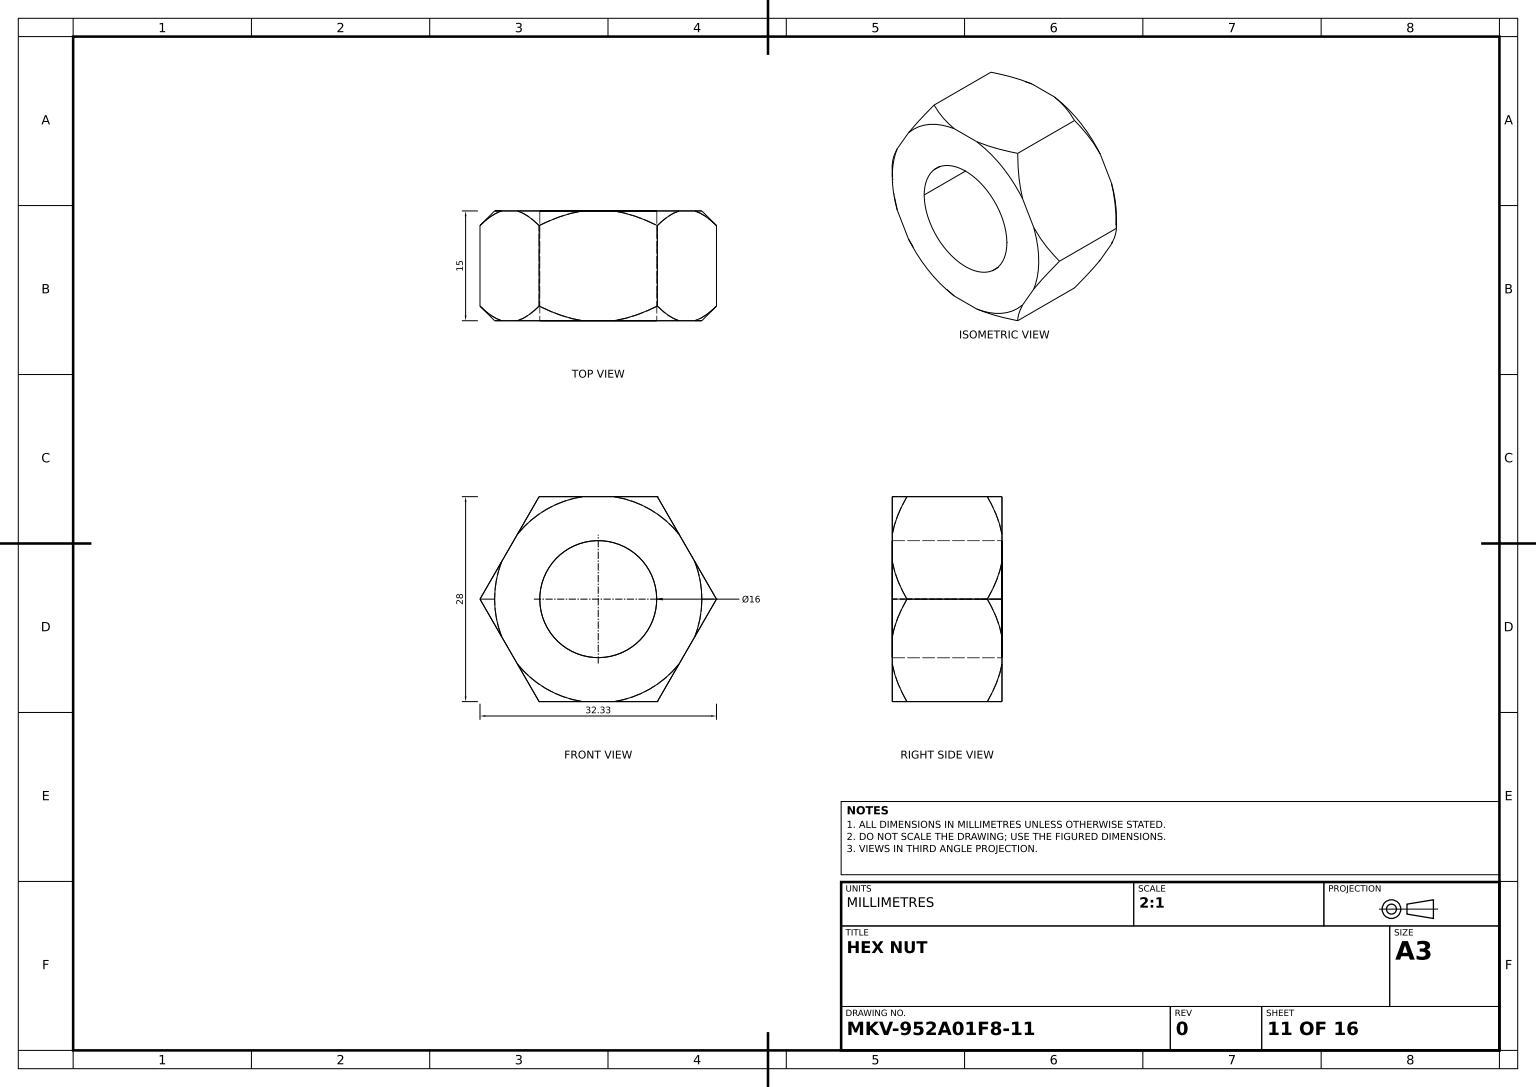
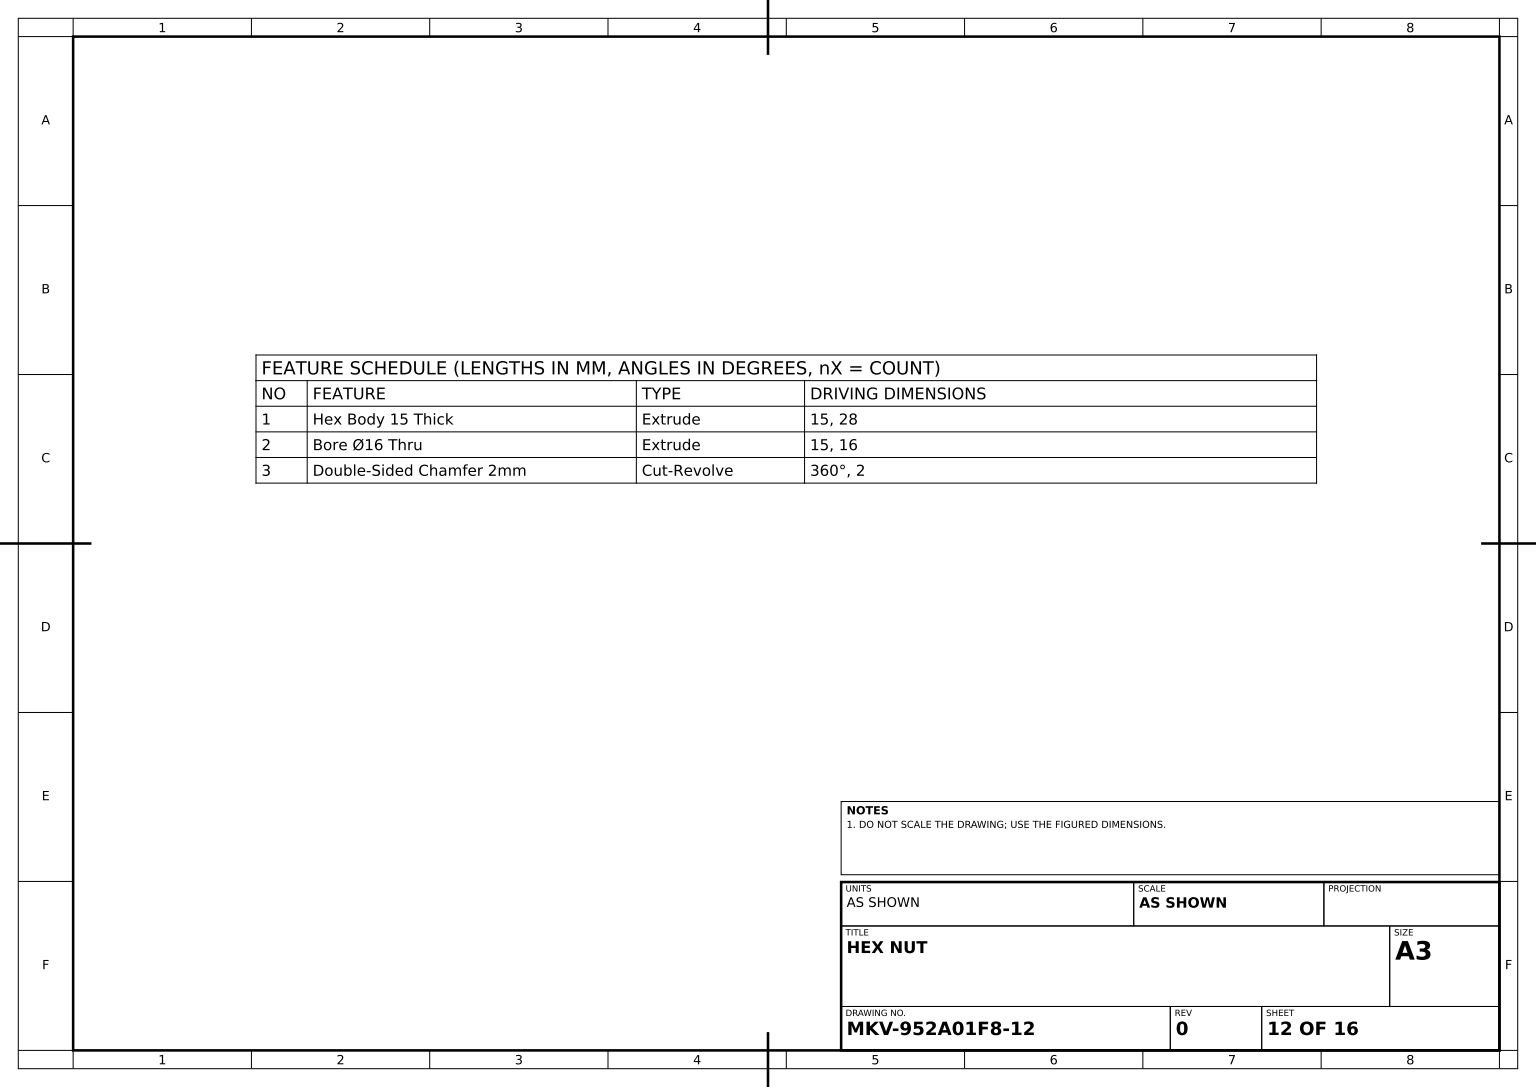
ISO-10303-21;
HEADER;
FILE_DESCRIPTION((''),'2;1');
FILE_NAME('','',(''),(''),'','','');
FILE_SCHEMA(('AUTOMOTIVE_DESIGN'));
ENDSEC;
DATA;
#1=APPLICATION_CONTEXT('');
#2=PRODUCT_CONTEXT('',#1,'mechanical');
#3=PRODUCT('','','',(#2));
#4=PRODUCT_DEFINITION_FORMATION('','',#3);
#5=PRODUCT_DEFINITION_CONTEXT('',#1,'design');
#6=PRODUCT_DEFINITION('','',#4,#5);
#7=PRODUCT_DEFINITION_SHAPE('','',#6);
#8=(LENGTH_UNIT()NAMED_UNIT(*)SI_UNIT(.MILLI.,.METRE.));
#9=(NAMED_UNIT(*)PLANE_ANGLE_UNIT()SI_UNIT($,.RADIAN.));
#10=(NAMED_UNIT(*)SI_UNIT($,.STERADIAN.)SOLID_ANGLE_UNIT());
#11=UNCERTAINTY_MEASURE_WITH_UNIT(LENGTH_MEASURE(1.E-05),#8,'distance_accuracy_value','');
#12=(GEOMETRIC_REPRESENTATION_CONTEXT(3)GLOBAL_UNCERTAINTY_ASSIGNED_CONTEXT((#11))GLOBAL_UNIT_ASSIGNED_CONTEXT((#8,#9,#10))REPRESENTATION_CONTEXT('',''));
#13=CARTESIAN_POINT('',(16.165808,0.,5.5));
#14=VERTEX_POINT('',#13);
#15=CARTESIAN_POINT('',(13.204877,-5.128483,7.5));
#16=VERTEX_POINT('',#15);
#17=CARTESIAN_POINT('',(15.693285,-0.818433,5.972523));
#18=CARTESIAN_POINT('',(15.212718,-1.6508,6.391638));
#19=CARTESIAN_POINT('',(14.228435,-3.355628,7.07619));
#20=CARTESIAN_POINT('',(13.724685,-4.228148,7.341403));
#21=B_SPLINE_CURVE_WITH_KNOTS('',3,(#13,#17,#18,#19,#20,#15),.UNSPECIFIED.,.F.,.F.,(4,2,4),(0.000000891,0.003124417,0.006247943),.UNSPECIFIED.);
#22=EDGE_CURVE('',#14,#16,#21,.T.);
#23=ORIENTED_EDGE('',*,*,#22,.T.);
#24=CARTESIAN_POINT('',(11.043835,-8.871517,7.5));
#25=VERTEX_POINT('',#24);
#26=CARTESIAN_POINT('',(8.082904,-14.,7.5));
#27=DIRECTION('',(0.5,0.866025404,0.));
#28=VECTOR('',#27,1000.);
#29=LINE('',#26,#28);
#30=EDGE_CURVE('',#25,#16,#29,.T.);
#31=ORIENTED_EDGE('',*,*,#30,.F.);
#32=CARTESIAN_POINT('',(8.082904,-14.,5.5));
#33=VERTEX_POINT('',#32);
#34=CARTESIAN_POINT('',(10.787509,-9.315486,7.421793));
#35=CARTESIAN_POINT('',(10.532672,-9.756876,7.316818));
#36=CARTESIAN_POINT('',(10.025695,-10.634987,7.058372));
#37=CARTESIAN_POINT('',(9.773626,-11.071583,6.904751));
#38=CARTESIAN_POINT('',(9.031896,-12.356297,6.388584));
#39=CARTESIAN_POINT('',(8.552376,-13.186851,5.969472));
#40=B_SPLINE_CURVE_WITH_KNOTS('',3,(#24,#34,#35,#36,#37,#38,#39,#32),.UNSPECIFIED.,.F.,.F.,(4,2,2,4),(0.010529143,0.012071736,0.013614329,0.016699514),.UNSPECIFIED.);
#41=EDGE_CURVE('',#25,#33,#40,.T.);
#42=ORIENTED_EDGE('',*,*,#41,.T.);
#43=CARTESIAN_POINT('',(8.082904,-14.,-5.5));
#44=VERTEX_POINT('',#43);
#45=DIRECTION('',(0.,0.,-1.));
#46=VECTOR('',#45,1000.);
#47=LINE('',#26,#46);
#48=EDGE_CURVE('',#33,#44,#47,.T.);
#49=ORIENTED_EDGE('',*,*,#48,.T.);
#50=CARTESIAN_POINT('',(11.043835,-8.871517,-7.5));
#51=VERTEX_POINT('',#50);
#52=CARTESIAN_POINT('',(8.555426,-13.181567,-5.972523));
#53=CARTESIAN_POINT('',(9.035994,-12.3492,-6.391638));
#54=CARTESIAN_POINT('',(10.020277,-10.644372,-7.07619));
#55=CARTESIAN_POINT('',(10.524026,-9.771852,-7.341403));
#56=B_SPLINE_CURVE_WITH_KNOTS('',3,(#43,#52,#53,#54,#55,#50),.UNSPECIFIED.,.F.,.F.,(4,2,4),(0.000000891,0.003124417,0.006247943),.UNSPECIFIED.);
#57=EDGE_CURVE('',#44,#51,#56,.T.);
#58=ORIENTED_EDGE('',*,*,#57,.T.);
#59=CARTESIAN_POINT('',(13.204877,-5.128483,-7.5));
#60=VERTEX_POINT('',#59);
#61=CARTESIAN_POINT('',(8.082904,-14.,-7.5));
#62=LINE('',#61,#28);
#63=EDGE_CURVE('',#51,#60,#62,.T.);
#64=ORIENTED_EDGE('',*,*,#63,.T.);
#65=CARTESIAN_POINT('',(16.165808,0.,-5.5));
#66=VERTEX_POINT('',#65);
#67=CARTESIAN_POINT('',(13.461202,-4.684514,-7.421793));
#68=CARTESIAN_POINT('',(13.716039,-4.243124,-7.316818));
#69=CARTESIAN_POINT('',(14.223016,-3.365013,-7.058372));
#70=CARTESIAN_POINT('',(14.475085,-2.928417,-6.904751));
#71=CARTESIAN_POINT('',(15.216815,-1.643703,-6.388584));
#72=CARTESIAN_POINT('',(15.696336,-0.813149,-5.969472));
#73=B_SPLINE_CURVE_WITH_KNOTS('',3,(#59,#67,#68,#69,#70,#71,#72,#65),.UNSPECIFIED.,.F.,.F.,(4,2,2,4),(0.010529143,0.012071736,0.013614329,0.016699514),.UNSPECIFIED.);
#74=EDGE_CURVE('',#60,#66,#73,.T.);
#75=ORIENTED_EDGE('',*,*,#74,.T.);
#76=CARTESIAN_POINT('',(16.165808,0.,7.5));
#77=LINE('',#76,#46);
#78=EDGE_CURVE('',#14,#66,#77,.T.);
#79=ORIENTED_EDGE('',*,*,#78,.F.);
#80=EDGE_LOOP('',(#23,#31,#42,#49,#58,#64,#75,#79));
#81=FACE_OUTER_BOUND('',#80,.T.);
#82=DIRECTION('',(-0.866025404,0.5,0.));
#83=DIRECTION('',(-0.5,-0.866025404,0.));
#84=AXIS2_PLACEMENT_3D('',#26,#82,#83);
#85=PLANE('',#84);
#86=ADVANCED_FACE('',(#81),#85,.F.);
#87=CARTESIAN_POINT('',(13.204877,5.128483,7.5));
#88=VERTEX_POINT('',#87);
#89=CARTESIAN_POINT('',(13.461202,4.684514,7.421793));
#90=CARTESIAN_POINT('',(13.716039,4.243124,7.316818));
#91=CARTESIAN_POINT('',(14.223016,3.365013,7.058372));
#92=CARTESIAN_POINT('',(14.475085,2.928417,6.904751));
#93=CARTESIAN_POINT('',(15.216815,1.643703,6.388584));
#94=CARTESIAN_POINT('',(15.696336,0.813149,5.969472));
#95=B_SPLINE_CURVE_WITH_KNOTS('',3,(#87,#89,#90,#91,#92,#93,#94,#13),.UNSPECIFIED.,.F.,.F.,(4,2,2,4),(0.010529143,0.012071736,0.013614329,0.016699514),.UNSPECIFIED.);
#96=EDGE_CURVE('',#88,#14,#95,.T.);
#97=ORIENTED_EDGE('',*,*,#96,.F.);
#98=CARTESIAN_POINT('',(0.,0.,7.5));
#99=DIRECTION('',(1.,0.,0.));
#100=AXIS2_PLACEMENT_3D('',#98,#45,#99);
#101=CIRCLE('',#100,14.165808);
#102=EDGE_CURVE('',#88,#16,#101,.T.);
#103=ORIENTED_EDGE('',*,*,#102,.T.);
#104=ORIENTED_EDGE('',*,*,#22,.F.);
#105=EDGE_LOOP('',(#97,#103,#104));
#106=FACE_OUTER_BOUND('',#105,.T.);
#107=CARTESIAN_POINT('',(0.,0.,5.5));
#108=DIRECTION('',(-1.,0.,0.));
#109=AXIS2_PLACEMENT_3D('',#107,#45,#108);
#110=CONICAL_SURFACE('',#109,16.165807537,0.785398163);
#111=ADVANCED_FACE('',(#106),#110,.T.);
#112=CARTESIAN_POINT('',(2.161042,-14.,-7.5));
#113=VERTEX_POINT('',#112);
#114=CARTESIAN_POINT('',(0.,0.,-7.5));
#115=AXIS2_PLACEMENT_3D('',#114,#45,#99);
#116=CIRCLE('',#115,14.165808);
#117=EDGE_CURVE('',#51,#113,#116,.T.);
#118=ORIENTED_EDGE('',*,*,#117,.F.);
#119=ORIENTED_EDGE('',*,*,#57,.F.);
#120=CARTESIAN_POINT('',(2.673693,-14.,-7.421793));
#121=CARTESIAN_POINT('',(3.183366,-14.,-7.316818));
#122=CARTESIAN_POINT('',(4.197321,-14.,-7.058372));
#123=CARTESIAN_POINT('',(4.701458,-14.,-6.904751));
#124=CARTESIAN_POINT('',(6.184918,-14.,-6.388584));
#125=CARTESIAN_POINT('',(7.14396,-14.,-5.969472));
#126=B_SPLINE_CURVE_WITH_KNOTS('',3,(#112,#120,#121,#122,#123,#124,#125,#43),.UNSPECIFIED.,.F.,.F.,(4,2,2,4),(0.010529025,0.012071618,0.013614211,0.016699398),.UNSPECIFIED.);
#127=EDGE_CURVE('',#113,#44,#126,.T.);
#128=ORIENTED_EDGE('',*,*,#127,.F.);
#129=EDGE_LOOP('',(#118,#119,#128));
#130=FACE_OUTER_BOUND('',#129,.T.);
#131=DIRECTION('',(0.,0.,1.));
#132=AXIS2_PLACEMENT_3D('',#114,#131,#99);
#133=CONICAL_SURFACE('',#132,14.165807537,0.785398163);
#134=ADVANCED_FACE('',(#130),#133,.T.);
#135=CARTESIAN_POINT('',(2.161042,14.,7.5));
#136=VERTEX_POINT('',#135);
#137=CARTESIAN_POINT('',(-2.161042,14.,7.5));
#138=VERTEX_POINT('',#137);
#139=CARTESIAN_POINT('',(8.082904,14.,7.5));
#140=VECTOR('',#108,1000.);
#141=LINE('',#139,#140);
#142=EDGE_CURVE('',#136,#138,#141,.T.);
#143=ORIENTED_EDGE('',*,*,#142,.F.);
#144=CARTESIAN_POINT('',(8.082904,14.,5.5));
#145=VERTEX_POINT('',#144);
#146=CARTESIAN_POINT('',(2.673693,14.,7.421793));
#147=CARTESIAN_POINT('',(3.183366,14.,7.316818));
#148=CARTESIAN_POINT('',(4.197321,14.,7.058372));
#149=CARTESIAN_POINT('',(4.701458,14.,6.904751));
#150=CARTESIAN_POINT('',(6.184918,14.,6.388584));
#151=CARTESIAN_POINT('',(7.14396,14.,5.969472));
#152=B_SPLINE_CURVE_WITH_KNOTS('',3,(#135,#146,#147,#148,#149,#150,#151,#144),.UNSPECIFIED.,.F.,.F.,(4,2,2,4),(0.010529025,0.012071618,0.013614211,0.016699398),.UNSPECIFIED.);
#153=EDGE_CURVE('',#136,#145,#152,.T.);
#154=ORIENTED_EDGE('',*,*,#153,.T.);
#155=CARTESIAN_POINT('',(8.082904,14.,-5.5));
#156=VERTEX_POINT('',#155);
#157=LINE('',#139,#46);
#158=EDGE_CURVE('',#145,#156,#157,.T.);
#159=ORIENTED_EDGE('',*,*,#158,.T.);
#160=CARTESIAN_POINT('',(2.161042,14.,-7.5));
#161=VERTEX_POINT('',#160);
#162=CARTESIAN_POINT('',(7.137858,14.,-5.972523));
#163=CARTESIAN_POINT('',(6.176723,14.,-6.391638));
#164=CARTESIAN_POINT('',(4.208157,14.,-7.07619));
#165=CARTESIAN_POINT('',(3.200659,14.,-7.341403));
#166=B_SPLINE_CURVE_WITH_KNOTS('',3,(#155,#162,#163,#164,#165,#160),.UNSPECIFIED.,.F.,.F.,(4,2,4),(0.000000771,0.003124297,0.006247823),.UNSPECIFIED.);
#167=EDGE_CURVE('',#156,#161,#166,.T.);
#168=ORIENTED_EDGE('',*,*,#167,.T.);
#169=CARTESIAN_POINT('',(-2.161042,14.,-7.5));
#170=VERTEX_POINT('',#169);
#171=CARTESIAN_POINT('',(8.082904,14.,-7.5));
#172=LINE('',#171,#140);
#173=EDGE_CURVE('',#161,#170,#172,.T.);
#174=ORIENTED_EDGE('',*,*,#173,.T.);
#175=CARTESIAN_POINT('',(-8.082904,14.,-5.5));
#176=VERTEX_POINT('',#175);
#177=CARTESIAN_POINT('',(-2.673693,14.,-7.421793));
#178=CARTESIAN_POINT('',(-3.183366,14.,-7.316818));
#179=CARTESIAN_POINT('',(-4.197321,14.,-7.058372));
#180=CARTESIAN_POINT('',(-4.701458,14.,-6.904751));
#181=CARTESIAN_POINT('',(-6.184918,14.,-6.388584));
#182=CARTESIAN_POINT('',(-7.14396,14.,-5.969472));
#183=B_SPLINE_CURVE_WITH_KNOTS('',3,(#169,#177,#178,#179,#180,#181,#182,#175),.UNSPECIFIED.,.F.,.F.,(4,2,2,4),(0.010529025,0.012071618,0.013614211,0.016699398),.UNSPECIFIED.);
#184=EDGE_CURVE('',#170,#176,#183,.T.);
#185=ORIENTED_EDGE('',*,*,#184,.T.);
#186=CARTESIAN_POINT('',(-8.082904,14.,5.5));
#187=VERTEX_POINT('',#186);
#188=CARTESIAN_POINT('',(-8.082904,14.,7.5));
#189=LINE('',#188,#46);
#190=EDGE_CURVE('',#187,#176,#189,.T.);
#191=ORIENTED_EDGE('',*,*,#190,.F.);
#192=CARTESIAN_POINT('',(-7.137858,14.,5.972523));
#193=CARTESIAN_POINT('',(-6.176723,14.,6.391638));
#194=CARTESIAN_POINT('',(-4.208157,14.,7.07619));
#195=CARTESIAN_POINT('',(-3.200659,14.,7.341403));
#196=B_SPLINE_CURVE_WITH_KNOTS('',3,(#186,#192,#193,#194,#195,#137),.UNSPECIFIED.,.F.,.F.,(4,2,4),(0.000000771,0.003124297,0.006247823),.UNSPECIFIED.);
#197=EDGE_CURVE('',#187,#138,#196,.T.);
#198=ORIENTED_EDGE('',*,*,#197,.T.);
#199=EDGE_LOOP('',(#143,#154,#159,#168,#174,#185,#191,#198));
#200=FACE_OUTER_BOUND('',#199,.T.);
#201=DIRECTION('',(0.,-1.,0.));
#202=AXIS2_PLACEMENT_3D('',#139,#201,#99);
#203=PLANE('',#202);
#204=ADVANCED_FACE('',(#200),#203,.F.);
#205=CARTESIAN_POINT('',(-14.165808,0.,7.5));
#206=VERTEX_POINT('',#205);
#207=CARTESIAN_POINT('',(-16.165808,0.,5.5));
#208=VERTEX_POINT('',#207);
#209=DIRECTION('',(-0.707106781,0.,-0.707106781));
#210=VECTOR('',#209,1000.);
#211=LINE('',#207,#210);
#212=EDGE_CURVE('',#206,#208,#211,.T.);
#213=ORIENTED_EDGE('',*,*,#212,.T.);
#214=CARTESIAN_POINT('',(-13.204877,-5.128483,7.5));
#215=VERTEX_POINT('',#214);
#216=CARTESIAN_POINT('',(-13.461202,-4.684514,7.421793));
#217=CARTESIAN_POINT('',(-13.716039,-4.243124,7.316818));
#218=CARTESIAN_POINT('',(-14.223016,-3.365013,7.058372));
#219=CARTESIAN_POINT('',(-14.475085,-2.928417,6.904751));
#220=CARTESIAN_POINT('',(-15.216815,-1.643703,6.388584));
#221=CARTESIAN_POINT('',(-15.696336,-0.813149,5.969472));
#222=B_SPLINE_CURVE_WITH_KNOTS('',3,(#214,#216,#217,#218,#219,#220,#221,#207),.UNSPECIFIED.,.F.,.F.,(4,2,2,4),(0.010529143,0.012071736,0.013614329,0.016699514),.UNSPECIFIED.);
#223=EDGE_CURVE('',#215,#208,#222,.T.);
#224=ORIENTED_EDGE('',*,*,#223,.F.);
#225=EDGE_CURVE('',#215,#206,#101,.T.);
#226=ORIENTED_EDGE('',*,*,#225,.T.);
#227=EDGE_LOOP('',(#213,#224,#226));
#228=FACE_OUTER_BOUND('',#227,.T.);
#229=ADVANCED_FACE('',(#228),#110,.T.);
#230=CARTESIAN_POINT('',(-8.,0.,-7.5));
#231=VERTEX_POINT('',#230);
#232=CARTESIAN_POINT('',(8.,0.,-7.5));
#233=VERTEX_POINT('',#232);
#234=CIRCLE('',#132,8.);
#235=EDGE_CURVE('',#231,#233,#234,.T.);
#236=ORIENTED_EDGE('',*,*,#235,.T.);
#237=EDGE_CURVE('',#233,#231,#234,.T.);
#238=ORIENTED_EDGE('',*,*,#237,.T.);
#239=EDGE_LOOP('',(#236,#238));
#240=FACE_BOUND('',#239,.T.);
#241=CARTESIAN_POINT('',(-2.161042,-14.,-7.5));
#242=VERTEX_POINT('',#241);
#243=CARTESIAN_POINT('',(-8.082904,-14.,-7.5));
#244=VECTOR('',#99,1000.);
#245=LINE('',#243,#244);
#246=EDGE_CURVE('',#242,#113,#245,.T.);
#247=ORIENTED_EDGE('',*,*,#246,.F.);
#248=CARTESIAN_POINT('',(-11.043835,-8.871517,-7.5));
#249=VERTEX_POINT('',#248);
#250=EDGE_CURVE('',#242,#249,#116,.T.);
#251=ORIENTED_EDGE('',*,*,#250,.T.);
#252=CARTESIAN_POINT('',(-13.204877,-5.128483,-7.5));
#253=VERTEX_POINT('',#252);
#254=CARTESIAN_POINT('',(-16.165808,0.,-7.5));
#255=DIRECTION('',(0.5,-0.866025404,0.));
#256=VECTOR('',#255,1000.);
#257=LINE('',#254,#256);
#258=EDGE_CURVE('',#253,#249,#257,.T.);
#259=ORIENTED_EDGE('',*,*,#258,.F.);
#260=CARTESIAN_POINT('',(-13.204877,5.128483,-7.5));
#261=VERTEX_POINT('',#260);
#262=EDGE_CURVE('',#253,#261,#116,.T.);
#263=ORIENTED_EDGE('',*,*,#262,.T.);
#264=CARTESIAN_POINT('',(-11.043835,8.871517,-7.5));
#265=VERTEX_POINT('',#264);
#266=CARTESIAN_POINT('',(-8.082904,14.,-7.5));
#267=VECTOR('',#83,1000.);
#268=LINE('',#266,#267);
#269=EDGE_CURVE('',#265,#261,#268,.T.);
#270=ORIENTED_EDGE('',*,*,#269,.F.);
#271=EDGE_CURVE('',#265,#170,#116,.T.);
#272=ORIENTED_EDGE('',*,*,#271,.T.);
#273=ORIENTED_EDGE('',*,*,#173,.F.);
#274=CARTESIAN_POINT('',(11.043835,8.871517,-7.5));
#275=VERTEX_POINT('',#274);
#276=EDGE_CURVE('',#161,#275,#116,.T.);
#277=ORIENTED_EDGE('',*,*,#276,.T.);
#278=CARTESIAN_POINT('',(13.204877,5.128483,-7.5));
#279=VERTEX_POINT('',#278);
#280=CARTESIAN_POINT('',(16.165808,0.,-7.5));
#281=DIRECTION('',(-0.5,0.866025404,0.));
#282=VECTOR('',#281,1000.);
#283=LINE('',#280,#282);
#284=EDGE_CURVE('',#279,#275,#283,.T.);
#285=ORIENTED_EDGE('',*,*,#284,.F.);
#286=CARTESIAN_POINT('',(14.165808,0.,-7.5));
#287=VERTEX_POINT('',#286);
#288=EDGE_CURVE('',#279,#287,#116,.T.);
#289=ORIENTED_EDGE('',*,*,#288,.T.);
#290=EDGE_CURVE('',#287,#60,#116,.T.);
#291=ORIENTED_EDGE('',*,*,#290,.T.);
#292=ORIENTED_EDGE('',*,*,#63,.F.);
#293=ORIENTED_EDGE('',*,*,#117,.T.);
#294=EDGE_LOOP('',(#247,#251,#259,#263,#270,#272,#273,#277,#285,#289,#291,#292,#293));
#295=FACE_OUTER_BOUND('',#294,.T.);
#296=PLANE('',#132);
#297=ADVANCED_FACE('',(#240,#295),#296,.F.);
#298=CARTESIAN_POINT('',(-11.043835,8.871517,7.5));
#299=VERTEX_POINT('',#298);
#300=CARTESIAN_POINT('',(-13.204877,5.128483,7.5));
#301=VERTEX_POINT('',#300);
#302=LINE('',#188,#267);
#303=EDGE_CURVE('',#299,#301,#302,.T.);
#304=ORIENTED_EDGE('',*,*,#303,.T.);
#305=EDGE_CURVE('',#206,#301,#101,.T.);
#306=ORIENTED_EDGE('',*,*,#305,.F.);
#307=ORIENTED_EDGE('',*,*,#225,.F.);
#308=CARTESIAN_POINT('',(-11.043835,-8.871517,7.5));
#309=VERTEX_POINT('',#308);
#310=CARTESIAN_POINT('',(-16.165808,0.,7.5));
#311=LINE('',#310,#256);
#312=EDGE_CURVE('',#215,#309,#311,.T.);
#313=ORIENTED_EDGE('',*,*,#312,.T.);
#314=CARTESIAN_POINT('',(-2.161042,-14.,7.5));
#315=VERTEX_POINT('',#314);
#316=EDGE_CURVE('',#315,#309,#101,.T.);
#317=ORIENTED_EDGE('',*,*,#316,.F.);
#318=CARTESIAN_POINT('',(2.161042,-14.,7.5));
#319=VERTEX_POINT('',#318);
#320=CARTESIAN_POINT('',(-8.082904,-14.,7.5));
#321=LINE('',#320,#244);
#322=EDGE_CURVE('',#315,#319,#321,.T.);
#323=ORIENTED_EDGE('',*,*,#322,.T.);
#324=EDGE_CURVE('',#25,#319,#101,.T.);
#325=ORIENTED_EDGE('',*,*,#324,.F.);
#326=ORIENTED_EDGE('',*,*,#30,.T.);
#327=ORIENTED_EDGE('',*,*,#102,.F.);
#328=CARTESIAN_POINT('',(11.043835,8.871517,7.5));
#329=VERTEX_POINT('',#328);
#330=LINE('',#76,#282);
#331=EDGE_CURVE('',#88,#329,#330,.T.);
#332=ORIENTED_EDGE('',*,*,#331,.T.);
#333=EDGE_CURVE('',#136,#329,#101,.T.);
#334=ORIENTED_EDGE('',*,*,#333,.F.);
#335=ORIENTED_EDGE('',*,*,#142,.T.);
#336=EDGE_CURVE('',#299,#138,#101,.T.);
#337=ORIENTED_EDGE('',*,*,#336,.F.);
#338=EDGE_LOOP('',(#304,#306,#307,#313,#317,#323,#325,#326,#327,#332,#334,#335,#337));
#339=FACE_OUTER_BOUND('',#338,.T.);
#340=CARTESIAN_POINT('',(-8.,0.,7.5));
#341=VERTEX_POINT('',#340);
#342=CARTESIAN_POINT('',(8.,0.,7.5));
#343=VERTEX_POINT('',#342);
#344=AXIS2_PLACEMENT_3D('',#98,#131,#99);
#345=CIRCLE('',#344,8.);
#346=EDGE_CURVE('',#341,#343,#345,.T.);
#347=ORIENTED_EDGE('',*,*,#346,.F.);
#348=EDGE_CURVE('',#343,#341,#345,.T.);
#349=ORIENTED_EDGE('',*,*,#348,.F.);
#350=EDGE_LOOP('',(#347,#349));
#351=FACE_BOUND('',#350,.T.);
#352=PLANE('',#344);
#353=ADVANCED_FACE('',(#339,#351),#352,.T.);
#354=ORIENTED_EDGE('',*,*,#322,.F.);
#355=CARTESIAN_POINT('',(-8.082904,-14.,5.5));
#356=VERTEX_POINT('',#355);
#357=CARTESIAN_POINT('',(-2.673693,-14.,7.421793));
#358=CARTESIAN_POINT('',(-3.183366,-14.,7.316818));
#359=CARTESIAN_POINT('',(-4.197321,-14.,7.058372));
#360=CARTESIAN_POINT('',(-4.701458,-14.,6.904751));
#361=CARTESIAN_POINT('',(-6.184918,-14.,6.388584));
#362=CARTESIAN_POINT('',(-7.14396,-14.,5.969472));
#363=B_SPLINE_CURVE_WITH_KNOTS('',3,(#314,#357,#358,#359,#360,#361,#362,#355),.UNSPECIFIED.,.F.,.F.,(4,2,2,4),(0.010529025,0.012071618,0.013614211,0.016699398),.UNSPECIFIED.);
#364=EDGE_CURVE('',#315,#356,#363,.T.);
#365=ORIENTED_EDGE('',*,*,#364,.T.);
#366=CARTESIAN_POINT('',(-8.082904,-14.,-5.5));
#367=VERTEX_POINT('',#366);
#368=LINE('',#320,#46);
#369=EDGE_CURVE('',#356,#367,#368,.T.);
#370=ORIENTED_EDGE('',*,*,#369,.T.);
#371=CARTESIAN_POINT('',(-7.137858,-14.,-5.972523));
#372=CARTESIAN_POINT('',(-6.176723,-14.,-6.391638));
#373=CARTESIAN_POINT('',(-4.208157,-14.,-7.07619));
#374=CARTESIAN_POINT('',(-3.200659,-14.,-7.341403));
#375=B_SPLINE_CURVE_WITH_KNOTS('',3,(#366,#371,#372,#373,#374,#241),.UNSPECIFIED.,.F.,.F.,(4,2,4),(0.000000771,0.003124297,0.006247823),.UNSPECIFIED.);
#376=EDGE_CURVE('',#367,#242,#375,.T.);
#377=ORIENTED_EDGE('',*,*,#376,.T.);
#378=ORIENTED_EDGE('',*,*,#246,.T.);
#379=ORIENTED_EDGE('',*,*,#127,.T.);
#380=ORIENTED_EDGE('',*,*,#48,.F.);
#381=CARTESIAN_POINT('',(7.137858,-14.,5.972523));
#382=CARTESIAN_POINT('',(6.176723,-14.,6.391638));
#383=CARTESIAN_POINT('',(4.208157,-14.,7.07619));
#384=CARTESIAN_POINT('',(3.200659,-14.,7.341403));
#385=B_SPLINE_CURVE_WITH_KNOTS('',3,(#32,#381,#382,#383,#384,#318),.UNSPECIFIED.,.F.,.F.,(4,2,4),(0.000000771,0.003124297,0.006247823),.UNSPECIFIED.);
#386=EDGE_CURVE('',#33,#319,#385,.T.);
#387=ORIENTED_EDGE('',*,*,#386,.T.);
#388=EDGE_LOOP('',(#354,#365,#370,#377,#378,#379,#380,#387));
#389=FACE_OUTER_BOUND('',#388,.T.);
#390=DIRECTION('',(0.,1.,0.));
#391=AXIS2_PLACEMENT_3D('',#320,#390,#108);
#392=PLANE('',#391);
#393=ADVANCED_FACE('',(#389),#392,.F.);
#394=ORIENTED_EDGE('',*,*,#364,.F.);
#395=ORIENTED_EDGE('',*,*,#316,.T.);
#396=CARTESIAN_POINT('',(-8.555426,-13.181567,5.972523));
#397=CARTESIAN_POINT('',(-9.035994,-12.3492,6.391638));
#398=CARTESIAN_POINT('',(-10.020277,-10.644372,7.07619));
#399=CARTESIAN_POINT('',(-10.524026,-9.771852,7.341403));
#400=B_SPLINE_CURVE_WITH_KNOTS('',3,(#355,#396,#397,#398,#399,#308),.UNSPECIFIED.,.F.,.F.,(4,2,4),(0.000000891,0.003124417,0.006247943),.UNSPECIFIED.);
#401=EDGE_CURVE('',#356,#309,#400,.T.);
#402=ORIENTED_EDGE('',*,*,#401,.F.);
#403=EDGE_LOOP('',(#394,#395,#402));
#404=FACE_OUTER_BOUND('',#403,.T.);
#405=ADVANCED_FACE('',(#404),#110,.T.);
#406=CARTESIAN_POINT('',(-15.693285,0.818433,5.972523));
#407=CARTESIAN_POINT('',(-15.212718,1.6508,6.391638));
#408=CARTESIAN_POINT('',(-14.228435,3.355628,7.07619));
#409=CARTESIAN_POINT('',(-13.724685,4.228148,7.341403));
#410=B_SPLINE_CURVE_WITH_KNOTS('',3,(#207,#406,#407,#408,#409,#300),.UNSPECIFIED.,.F.,.F.,(4,2,4),(0.000000891,0.003124417,0.006247943),.UNSPECIFIED.);
#411=EDGE_CURVE('',#208,#301,#410,.T.);
#412=ORIENTED_EDGE('',*,*,#411,.T.);
#413=ORIENTED_EDGE('',*,*,#303,.F.);
#414=CARTESIAN_POINT('',(-10.787509,9.315486,7.421793));
#415=CARTESIAN_POINT('',(-10.532672,9.756876,7.316818));
#416=CARTESIAN_POINT('',(-10.025695,10.634987,7.058372));
#417=CARTESIAN_POINT('',(-9.773626,11.071583,6.904751));
#418=CARTESIAN_POINT('',(-9.031896,12.356297,6.388584));
#419=CARTESIAN_POINT('',(-8.552376,13.186851,5.969472));
#420=B_SPLINE_CURVE_WITH_KNOTS('',3,(#298,#414,#415,#416,#417,#418,#419,#186),.UNSPECIFIED.,.F.,.F.,(4,2,2,4),(0.010529143,0.012071736,0.013614329,0.016699514),.UNSPECIFIED.);
#421=EDGE_CURVE('',#299,#187,#420,.T.);
#422=ORIENTED_EDGE('',*,*,#421,.T.);
#423=ORIENTED_EDGE('',*,*,#190,.T.);
#424=CARTESIAN_POINT('',(-8.555426,13.181567,-5.972523));
#425=CARTESIAN_POINT('',(-9.035994,12.3492,-6.391638));
#426=CARTESIAN_POINT('',(-10.020277,10.644372,-7.07619));
#427=CARTESIAN_POINT('',(-10.524026,9.771852,-7.341403));
#428=B_SPLINE_CURVE_WITH_KNOTS('',3,(#175,#424,#425,#426,#427,#264),.UNSPECIFIED.,.F.,.F.,(4,2,4),(0.000000891,0.003124417,0.006247943),.UNSPECIFIED.);
#429=EDGE_CURVE('',#176,#265,#428,.T.);
#430=ORIENTED_EDGE('',*,*,#429,.T.);
#431=ORIENTED_EDGE('',*,*,#269,.T.);
#432=CARTESIAN_POINT('',(-16.165808,0.,-5.5));
#433=VERTEX_POINT('',#432);
#434=CARTESIAN_POINT('',(-13.461202,4.684514,-7.421793));
#435=CARTESIAN_POINT('',(-13.716039,4.243124,-7.316818));
#436=CARTESIAN_POINT('',(-14.223016,3.365013,-7.058372));
#437=CARTESIAN_POINT('',(-14.475085,2.928417,-6.904751));
#438=CARTESIAN_POINT('',(-15.216815,1.643703,-6.388584));
#439=CARTESIAN_POINT('',(-15.696336,0.813149,-5.969472));
#440=B_SPLINE_CURVE_WITH_KNOTS('',3,(#260,#434,#435,#436,#437,#438,#439,#432),.UNSPECIFIED.,.F.,.F.,(4,2,2,4),(0.010529143,0.012071736,0.013614329,0.016699514),.UNSPECIFIED.);
#441=EDGE_CURVE('',#261,#433,#440,.T.);
#442=ORIENTED_EDGE('',*,*,#441,.T.);
#443=LINE('',#310,#46);
#444=EDGE_CURVE('',#208,#433,#443,.T.);
#445=ORIENTED_EDGE('',*,*,#444,.F.);
#446=EDGE_LOOP('',(#412,#413,#422,#423,#430,#431,#442,#445));
#447=FACE_OUTER_BOUND('',#446,.T.);
#448=DIRECTION('',(0.866025404,-0.5,0.));
#449=AXIS2_PLACEMENT_3D('',#188,#448,#27);
#450=PLANE('',#449);
#451=ADVANCED_FACE('',(#447),#450,.F.);
#452=VECTOR('',#131,1000.);
#453=LINE('',#232,#452);
#454=EDGE_CURVE('',#233,#343,#453,.T.);
#455=ORIENTED_EDGE('',*,*,#454,.T.);
#456=ORIENTED_EDGE('',*,*,#348,.T.);
#457=LINE('',#230,#452);
#458=EDGE_CURVE('',#231,#341,#457,.T.);
#459=ORIENTED_EDGE('',*,*,#458,.F.);
#460=ORIENTED_EDGE('',*,*,#237,.F.);
#461=EDGE_LOOP('',(#455,#456,#459,#460));
#462=FACE_OUTER_BOUND('',#461,.T.);
#463=CYLINDRICAL_SURFACE('',#132,8.);
#464=ADVANCED_FACE('',(#462),#463,.F.);
#465=ORIENTED_EDGE('',*,*,#369,.F.);
#466=ORIENTED_EDGE('',*,*,#401,.T.);
#467=ORIENTED_EDGE('',*,*,#312,.F.);
#468=ORIENTED_EDGE('',*,*,#223,.T.);
#469=ORIENTED_EDGE('',*,*,#444,.T.);
#470=CARTESIAN_POINT('',(-15.693285,-0.818433,-5.972523));
#471=CARTESIAN_POINT('',(-15.212718,-1.6508,-6.391638));
#472=CARTESIAN_POINT('',(-14.228435,-3.355628,-7.07619));
#473=CARTESIAN_POINT('',(-13.724685,-4.228148,-7.341403));
#474=B_SPLINE_CURVE_WITH_KNOTS('',3,(#432,#470,#471,#472,#473,#252),.UNSPECIFIED.,.F.,.F.,(4,2,4),(0.000000891,0.003124417,0.006247943),.UNSPECIFIED.);
#475=EDGE_CURVE('',#433,#253,#474,.T.);
#476=ORIENTED_EDGE('',*,*,#475,.T.);
#477=ORIENTED_EDGE('',*,*,#258,.T.);
#478=CARTESIAN_POINT('',(-10.787509,-9.315486,-7.421793));
#479=CARTESIAN_POINT('',(-10.532672,-9.756876,-7.316818));
#480=CARTESIAN_POINT('',(-10.025695,-10.634987,-7.058372));
#481=CARTESIAN_POINT('',(-9.773626,-11.071583,-6.904751));
#482=CARTESIAN_POINT('',(-9.031896,-12.356297,-6.388584));
#483=CARTESIAN_POINT('',(-8.552376,-13.186851,-5.969472));
#484=B_SPLINE_CURVE_WITH_KNOTS('',3,(#248,#478,#479,#480,#481,#482,#483,#366),.UNSPECIFIED.,.F.,.F.,(4,2,2,4),(0.010529143,0.012071736,0.013614329,0.016699514),.UNSPECIFIED.);
#485=EDGE_CURVE('',#249,#367,#484,.T.);
#486=ORIENTED_EDGE('',*,*,#485,.T.);
#487=EDGE_LOOP('',(#465,#466,#467,#468,#469,#476,#477,#486));
#488=FACE_OUTER_BOUND('',#487,.T.);
#489=DIRECTION('',(0.866025404,0.5,0.));
#490=AXIS2_PLACEMENT_3D('',#310,#489,#281);
#491=PLANE('',#490);
#492=ADVANCED_FACE('',(#488),#491,.F.);
#493=ORIENTED_EDGE('',*,*,#411,.F.);
#494=ORIENTED_EDGE('',*,*,#212,.F.);
#495=ORIENTED_EDGE('',*,*,#305,.T.);
#496=EDGE_LOOP('',(#493,#494,#495));
#497=FACE_OUTER_BOUND('',#496,.T.);
#498=ADVANCED_FACE('',(#497),#110,.T.);
#499=CARTESIAN_POINT('',(15.693285,0.818433,-5.972523));
#500=CARTESIAN_POINT('',(15.212718,1.6508,-6.391638));
#501=CARTESIAN_POINT('',(14.228435,3.355628,-7.07619));
#502=CARTESIAN_POINT('',(13.724685,4.228148,-7.341403));
#503=B_SPLINE_CURVE_WITH_KNOTS('',3,(#65,#499,#500,#501,#502,#278),.UNSPECIFIED.,.F.,.F.,(4,2,4),(0.000000891,0.003124417,0.006247943),.UNSPECIFIED.);
#504=EDGE_CURVE('',#66,#279,#503,.T.);
#505=ORIENTED_EDGE('',*,*,#504,.T.);
#506=ORIENTED_EDGE('',*,*,#284,.T.);
#507=CARTESIAN_POINT('',(10.787509,9.315486,-7.421793));
#508=CARTESIAN_POINT('',(10.532672,9.756876,-7.316818));
#509=CARTESIAN_POINT('',(10.025695,10.634987,-7.058372));
#510=CARTESIAN_POINT('',(9.773626,11.071583,-6.904751));
#511=CARTESIAN_POINT('',(9.031896,12.356297,-6.388584));
#512=CARTESIAN_POINT('',(8.552376,13.186851,-5.969472));
#513=B_SPLINE_CURVE_WITH_KNOTS('',3,(#274,#507,#508,#509,#510,#511,#512,#155),.UNSPECIFIED.,.F.,.F.,(4,2,2,4),(0.010529143,0.012071736,0.013614329,0.016699514),.UNSPECIFIED.);
#514=EDGE_CURVE('',#275,#156,#513,.T.);
#515=ORIENTED_EDGE('',*,*,#514,.T.);
#516=ORIENTED_EDGE('',*,*,#158,.F.);
#517=CARTESIAN_POINT('',(8.555426,13.181567,5.972523));
#518=CARTESIAN_POINT('',(9.035994,12.3492,6.391638));
#519=CARTESIAN_POINT('',(10.020277,10.644372,7.07619));
#520=CARTESIAN_POINT('',(10.524026,9.771852,7.341403));
#521=B_SPLINE_CURVE_WITH_KNOTS('',3,(#144,#517,#518,#519,#520,#328),.UNSPECIFIED.,.F.,.F.,(4,2,4),(0.000000891,0.003124417,0.006247943),.UNSPECIFIED.);
#522=EDGE_CURVE('',#145,#329,#521,.T.);
#523=ORIENTED_EDGE('',*,*,#522,.T.);
#524=ORIENTED_EDGE('',*,*,#331,.F.);
#525=ORIENTED_EDGE('',*,*,#96,.T.);
#526=ORIENTED_EDGE('',*,*,#78,.T.);
#527=EDGE_LOOP('',(#505,#506,#515,#516,#523,#524,#525,#526));
#528=FACE_OUTER_BOUND('',#527,.T.);
#529=DIRECTION('',(-0.866025404,-0.5,0.));
#530=AXIS2_PLACEMENT_3D('',#76,#529,#255);
#531=PLANE('',#530);
#532=ADVANCED_FACE('',(#528),#531,.F.);
#533=ORIENTED_EDGE('',*,*,#333,.T.);
#534=ORIENTED_EDGE('',*,*,#522,.F.);
#535=ORIENTED_EDGE('',*,*,#153,.F.);
#536=EDGE_LOOP('',(#533,#534,#535));
#537=FACE_OUTER_BOUND('',#536,.T.);
#538=ADVANCED_FACE('',(#537),#110,.T.);
#539=ORIENTED_EDGE('',*,*,#262,.F.);
#540=ORIENTED_EDGE('',*,*,#475,.F.);
#541=ORIENTED_EDGE('',*,*,#441,.F.);
#542=EDGE_LOOP('',(#539,#540,#541));
#543=FACE_OUTER_BOUND('',#542,.T.);
#544=ADVANCED_FACE('',(#543),#133,.T.);
#545=DIRECTION('',(0.707106781,0.,0.707106781));
#546=VECTOR('',#545,1000.);
#547=LINE('',#286,#546);
#548=EDGE_CURVE('',#287,#66,#547,.T.);
#549=ORIENTED_EDGE('',*,*,#548,.F.);
#550=ORIENTED_EDGE('',*,*,#288,.F.);
#551=ORIENTED_EDGE('',*,*,#504,.F.);
#552=EDGE_LOOP('',(#549,#550,#551));
#553=FACE_OUTER_BOUND('',#552,.T.);
#554=ADVANCED_FACE('',(#553),#133,.T.);
#555=ORIENTED_EDGE('',*,*,#548,.T.);
#556=ORIENTED_EDGE('',*,*,#74,.F.);
#557=ORIENTED_EDGE('',*,*,#290,.F.);
#558=EDGE_LOOP('',(#555,#556,#557));
#559=FACE_OUTER_BOUND('',#558,.T.);
#560=ADVANCED_FACE('',(#559),#133,.T.);
#561=ORIENTED_EDGE('',*,*,#41,.F.);
#562=ORIENTED_EDGE('',*,*,#324,.T.);
#563=ORIENTED_EDGE('',*,*,#386,.F.);
#564=EDGE_LOOP('',(#561,#562,#563));
#565=FACE_OUTER_BOUND('',#564,.T.);
#566=ADVANCED_FACE('',(#565),#110,.T.);
#567=ORIENTED_EDGE('',*,*,#458,.T.);
#568=ORIENTED_EDGE('',*,*,#346,.T.);
#569=ORIENTED_EDGE('',*,*,#454,.F.);
#570=ORIENTED_EDGE('',*,*,#235,.F.);
#571=EDGE_LOOP('',(#567,#568,#569,#570));
#572=FACE_OUTER_BOUND('',#571,.T.);
#573=ADVANCED_FACE('',(#572),#463,.F.);
#574=ORIENTED_EDGE('',*,*,#336,.T.);
#575=ORIENTED_EDGE('',*,*,#197,.F.);
#576=ORIENTED_EDGE('',*,*,#421,.F.);
#577=EDGE_LOOP('',(#574,#575,#576));
#578=FACE_OUTER_BOUND('',#577,.T.);
#579=ADVANCED_FACE('',(#578),#110,.T.);
#580=ORIENTED_EDGE('',*,*,#271,.F.);
#581=ORIENTED_EDGE('',*,*,#429,.F.);
#582=ORIENTED_EDGE('',*,*,#184,.F.);
#583=EDGE_LOOP('',(#580,#581,#582));
#584=FACE_OUTER_BOUND('',#583,.T.);
#585=ADVANCED_FACE('',(#584),#133,.T.);
#586=ORIENTED_EDGE('',*,*,#250,.F.);
#587=ORIENTED_EDGE('',*,*,#376,.F.);
#588=ORIENTED_EDGE('',*,*,#485,.F.);
#589=EDGE_LOOP('',(#586,#587,#588));
#590=FACE_OUTER_BOUND('',#589,.T.);
#591=ADVANCED_FACE('',(#590),#133,.T.);
#592=ORIENTED_EDGE('',*,*,#276,.F.);
#593=ORIENTED_EDGE('',*,*,#167,.F.);
#594=ORIENTED_EDGE('',*,*,#514,.F.);
#595=EDGE_LOOP('',(#592,#593,#594));
#596=FACE_OUTER_BOUND('',#595,.T.);
#597=ADVANCED_FACE('',(#596),#133,.T.);
#598=CLOSED_SHELL('',(#86,#111,#134,#204,#229,#297,#353,#393,#405,#451,#464,#492,#498,#532,#538,#544,#554,#560,#566,#573,#579,#585,#591,#597));
#599=MANIFOLD_SOLID_BREP('',#598);
#600=ADVANCED_BREP_SHAPE_REPRESENTATION('',(#599),#12);
#601=SHAPE_DEFINITION_REPRESENTATION(#7,#600);
ENDSEC;
END-ISO-10303-21;
